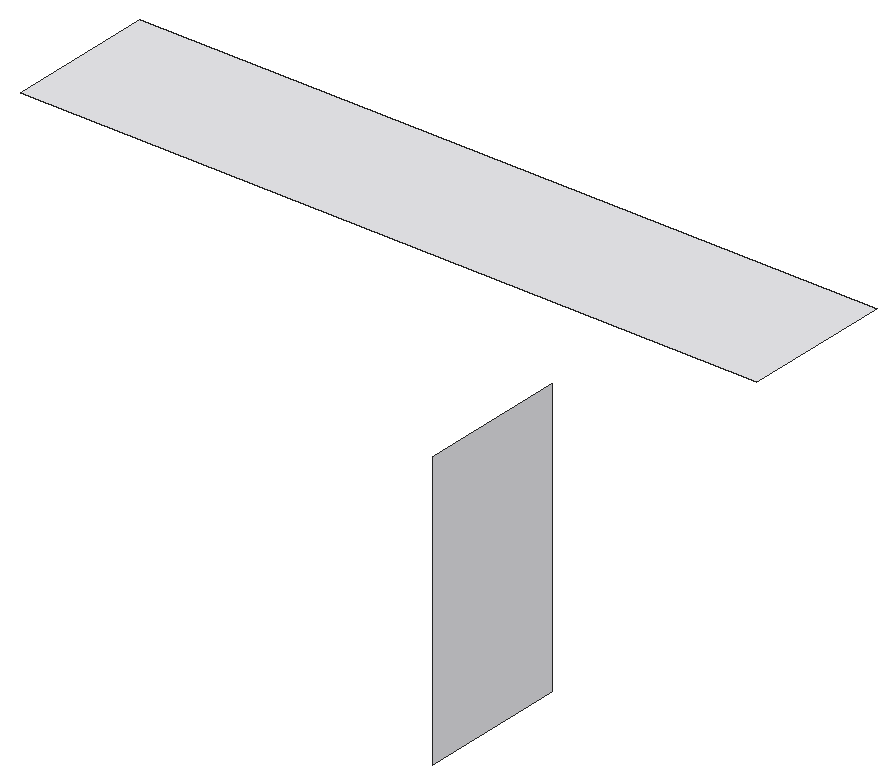
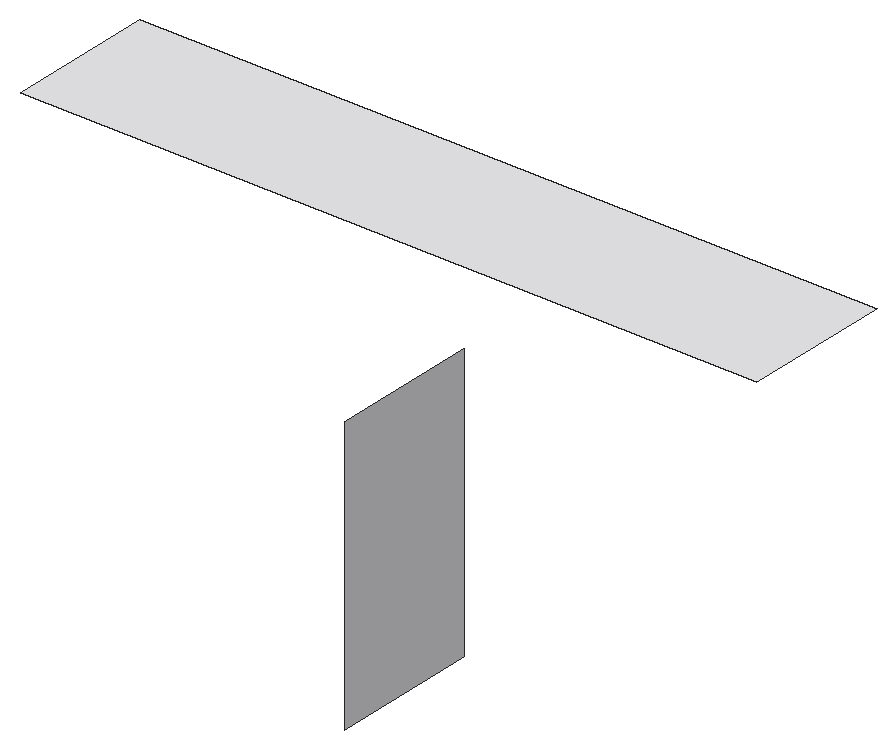
# SketchUp Ruby script. Lengths in inches.
U = 1.inch
M = Sketchup.active_model
def pt(a) = Geom::Point3d.new(a.map { |v| v * U })
def face(e, loops, mat)
  f = e.add_face(loops[0].map { |a| pt(a) })
  loops[1..].each { |l| e.add_face(l.map { |a| pt(a) }).erase! }
  f.material = f.back_material = mat if mat
  f
end
# faces: each face lists its corners as indices into pts; further lists are holes
def faces(e, pts, list, mat = nil) = list.each { |f| face(e, (f[0].is_a?(Array) ? f : [f]).map { |l| l.map { |i| pts[i] } }, mat) }
# xy, xz, yz: faces in a plane at the given z, y or x. An outline is a flat list of corners, or four numbers for a rectangle; further outlines are holes
def ring(l) = l.size == 4 ? [[l[0], l[1]], [l[2], l[1]], [l[2], l[3]], [l[0], l[3]]] : l.each_slice(2).to_a
def flat(e, list, mat, &to3) = list.each { |f| face(e, (f[0].is_a?(Array) ? f : [f]).map { |l| ring(l).map { |u, v| to3.(u, v) } }, mat) }
def xy(e, z, list, mat = nil) = flat(e, list, mat) { |x, y| [x, y, z] }
def xz(e, y, list, mat = nil) = flat(e, list, mat) { |x, z| [x, y, z] }
def yz(e, x, list, mat = nil) = flat(e, list, mat) { |y, z| [x, y, z] }
def lines(e, pts, list) = list.each { |a, b| e.add_line(pt(pts[a]), pt(pts[b])) }
# prism: a flat outline (further loops are holes) pulled along v
def prism(e, loops, v, mat = nil)
  f = face(e, loops, mat); d = Geom::Vector3d.new(v.map { |x| x * U })
  f.pushpull(f.normal.samedirection?(d) ? d.length : -d.length)
end
def box(e, o, s, mat = nil) = prism(e, [[o, [o[0] + s[0], o[1], o[2]], [o[0] + s[0], o[1] + s[1], o[2]], [o[0], o[1] + s[1], o[2]]]], [0, 0, s[2]], mat)
def at(x, y, z, deg = 0) = Geom::Transformation.translation(pt([x, y, z])) * Geom::Transformation.rotation(ORIGIN, Z_AXIS, deg.degrees)
def axes(o, x, y, z) = Geom::Transformation.new([*x, 0, *y, 0, *z, 0, *pt(o).to_a, 1])
def part(name) = M.definitions.add(name)
# library, detail: a bought-in or finely detailed component or shape, given as its bounding box
def library(name, o, s) = part(name).tap { |d| box(d.entities, o, s) }
def detail(e, o, s) = box(e.add_group.entities, o, s)
def put(e, d, t, mat = nil) = e.add_instance(d, t).tap { |i| i.material = mat if mat }
def group(e, t, mat = nil) = e.add_group.tap { |g| g.transformation = t; g.material = mat if mat }.entities
root = M.entities
M.materials.add("[Blinds Vertical Pattern]1").color = [239, 239, 242]
xy(root,52.34,[[213.78,96.24,286.85,111]],"[Blinds Vertical Pattern]1")
yz(root,254.71,[[96.24,7.1,111,34.41]],"[Blinds Vertical Pattern]1")
